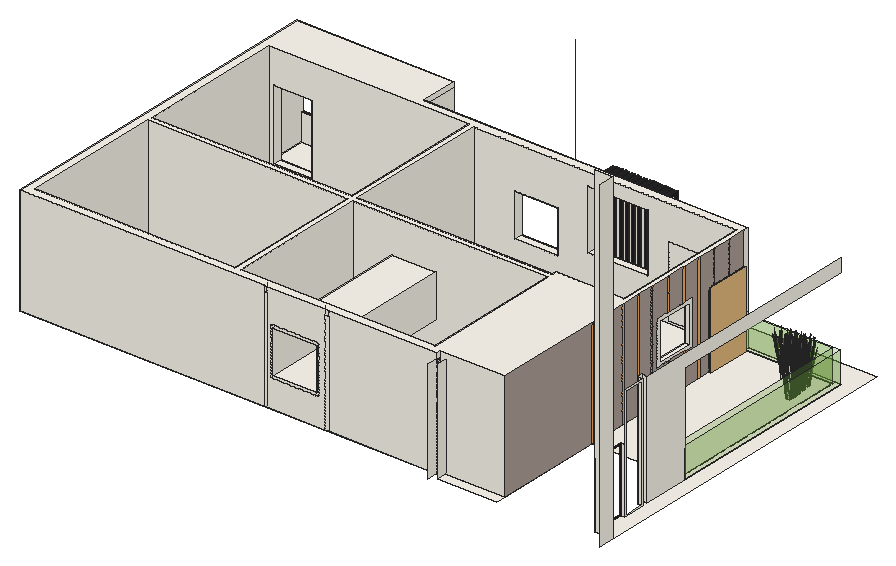
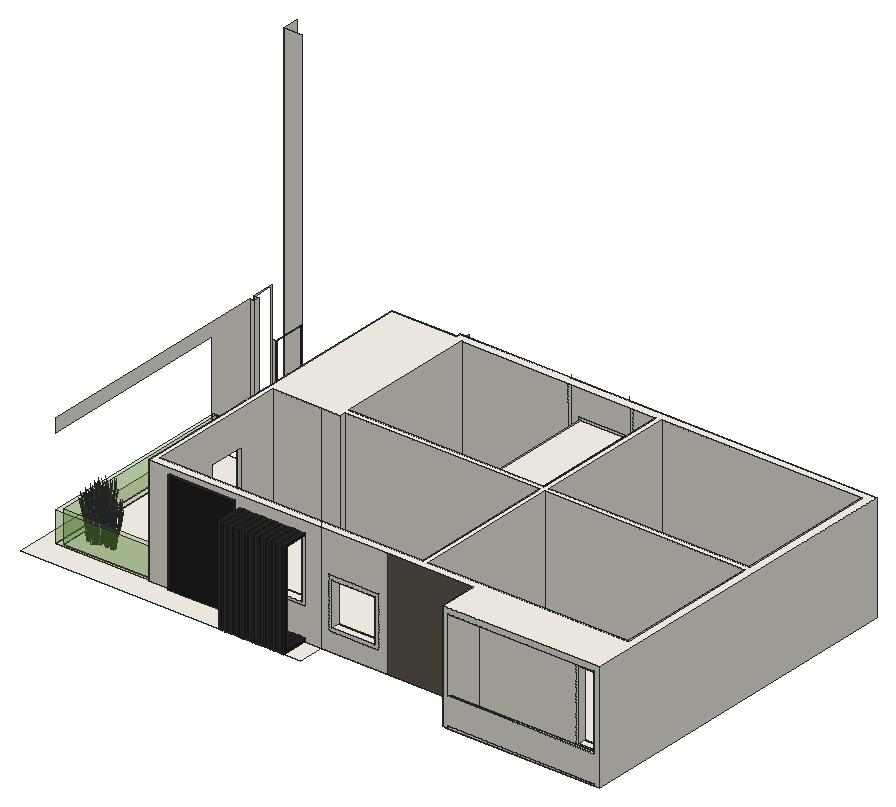
# SketchUp Ruby script. Lengths in inches.
U = 1.inch
M = Sketchup.active_model
def pt(a) = Geom::Point3d.new(a.map { |v| v * U })
def face(e, loops, mat)
  f = e.add_face(loops[0].map { |a| pt(a) })
  loops[1..].each { |l| e.add_face(l.map { |a| pt(a) }).erase! }
  f.material = f.back_material = mat if mat
  f
end
# faces: each face lists its corners as indices into pts; further lists are holes
def faces(e, pts, list, mat = nil) = list.each { |f| face(e, (f[0].is_a?(Array) ? f : [f]).map { |l| l.map { |i| pts[i] } }, mat) }
# xy, xz, yz: faces in a plane at the given z, y or x. An outline is a flat list of corners, or four numbers for a rectangle; further outlines are holes
def ring(l) = l.size == 4 ? [[l[0], l[1]], [l[2], l[1]], [l[2], l[3]], [l[0], l[3]]] : l.each_slice(2).to_a
def flat(e, list, mat, &to3) = list.each { |f| face(e, (f[0].is_a?(Array) ? f : [f]).map { |l| ring(l).map { |u, v| to3.(u, v) } }, mat) }
def xy(e, z, list, mat = nil) = flat(e, list, mat) { |x, y| [x, y, z] }
def xz(e, y, list, mat = nil) = flat(e, list, mat) { |x, z| [x, y, z] }
def yz(e, x, list, mat = nil) = flat(e, list, mat) { |y, z| [x, y, z] }
def lines(e, pts, list) = list.each { |a, b| e.add_line(pt(pts[a]), pt(pts[b])) }
# prism: a flat outline (further loops are holes) pulled along v
def prism(e, loops, v, mat = nil)
  f = face(e, loops, mat); d = Geom::Vector3d.new(v.map { |x| x * U })
  f.pushpull(f.normal.samedirection?(d) ? d.length : -d.length)
end
def box(e, o, s, mat = nil) = prism(e, [[o, [o[0] + s[0], o[1], o[2]], [o[0] + s[0], o[1] + s[1], o[2]], [o[0], o[1] + s[1], o[2]]]], [0, 0, s[2]], mat)
def at(x, y, z, deg = 0) = Geom::Transformation.translation(pt([x, y, z])) * Geom::Transformation.rotation(ORIGIN, Z_AXIS, deg.degrees)
def axes(o, x, y, z) = Geom::Transformation.new([*x, 0, *y, 0, *z, 0, *pt(o).to_a, 1])
def part(name) = M.definitions.add(name)
# library, detail: a bought-in or finely detailed component or shape, given as its bounding box
def library(name, o, s) = part(name).tap { |d| box(d.entities, o, s) }
def detail(e, o, s) = box(e.add_group.entities, o, s)
def put(e, d, t, mat = nil) = e.add_instance(d, t).tap { |i| i.material = mat if mat }
def group(e, t, mat = nil) = e.add_group.tap { |g| g.transformation = t; g.material = mat if mat }.entities
root = M.entities
M.materials.add("C01_Vanilla_Cream").color = [255, 251, 241]
M.materials.add("C03_Honey_Glow").color = [255, 178, 101]
M.materials.add("Glass_Basic_01").color = [119, 186, 61]
M.materials["Glass_Basic_01"].alpha = 0.25
M.materials.add("LightPink_Translucent").color = [144, 107, 117]
M.materials["LightPink_Translucent"].alpha = 0.75
M.materials.add("Marble_07_1K").color = [36, 34, 36]
M.materials.add("Plaster_04_1K").color = [106, 98, 87]
M.materials.add("ThomThom - Hair1").color = [178, 163, 155]
c1 = library("porta+4",[0.2,-5.42,1.33],[46.55,4.72,83.21])
c2 = part("blade")
p = [[2.15,0.21,22],[0,0.17,0],[0.09,0.45,0],[2.18,0.31,22],[2.29,0.31,22],[0.38,0.45,0],
  [2.48,0.24,33],[2.49,0.24,33],[2.48,0.22,33]]
faces(c2.entities,p,[[0,1,2,3],[4,5,2,3],[6,3,4,7],[8,0,3,6]])
c3 = part("seeds")
p = [[0.3,-0.1,1.38],[-0.01,-0.03,1.59],[-0.01,-0.03,0.03],[0.14,-0.07,-0.07],[0.29,-0.03,3],[0.15,0.01,3.11]]
faces(c3.entities,p,[[0,1,2,3],[1,0,4,5]],"LightPink_Translucent")
c4 = part("blade with seeds")
put(c4.entities,c2,at(0,0,0))
put(c4.entities,c3,axes([2.4,0.25,30.99],[1.5799,-0.05474,1.17369],[-0.12525,1.92788,0.29478],[-0.07173,-0.02425,1.56792]))
xy(root,264,[[537,12,603,24],[69,18,531,18,531,24,603,24,603,360,243,360,243,402,69,402],[702,24,722,24,722,389.16,411,389.16,411,360,706,360,706,91.21,700,91.21,700,85.38,706,85.38,706,60,702,60],[603,144,699.71,356],[699.71,144,706,360],
  [603,356,699.71,360]],"C01_Vanilla_Cream")
xz(root,24,[[531,264,537,378],[702,264,722,624]],"C01_Vanilla_Cream")
xz(root,60,[[702,264,706,336]],"C01_Vanilla_Cream")
xz(root,85.38,[[700,264,706,390]],"C01_Vanilla_Cream")
xz(root,91.21,[[700,264,706,390]],"C01_Vanilla_Cream")
xz(root,144,[[693.41,264,699.71,300],[699.71,264,706,300]],"C01_Vanilla_Cream")
xz(root,356,[[603,264,699.71,300]],"Glass_Basic_01")
xz(root,360,[[603,264,706,298]],"Glass_Basic_01")
yz(root,531,[[6,264,24,378]],"C01_Vanilla_Cream")
yz(root,537,[[12,264,24,378]],"C01_Vanilla_Cream")
yz(root,603,[[356,264,360,300]],"C01_Vanilla_Cream")
yz(root,699.71,[[144,264,356,300]],"Glass_Basic_01")
yz(root,700,[[85.38,264,91.21,390]],"C01_Vanilla_Cream")
yz(root,702,[[[24,264,60,336],[25,265,59,335]]],"Marble_07_1K")
yz(root,706,[[[60,264,85.38,390],[61,265,84.38,389]],[91.21,264,144,264,144,375,360,375,360,390,91.21,390]],"C01_Vanilla_Cream")
yz(root,706,[[144,264,360,298]],"Glass_Basic_01")
yz(root,722,[[6,264,24,624]],"C01_Vanilla_Cream")
p = [[411,360,504],[411,360,264]]
lines(root,p,[[0,1]])
put(root,c1,axes([599.84,305.79,262.64],[0,1.03118,0],[-1,0,0],[0,0,1.00971]))
g1 = group(root,at(69,18,264),"C01_Vanilla_Cream")
xy(g1,0,[[[0,0,0,384,6,384,6,342,168,342,168,384,174,384,174,342,360.88,342,360.88,371.16,364.88,371.16,364.88,342,367.67,342,367.67,371.16,371.67,371.16,371.67,342,374.46,342,374.46,371.16,378.46,371.16,378.46,342,381.25,342,381.25,371.16,385.25,371.16,385.25,342,388.04,342,388.04,371.16,392.04,371.16,392.04,342,394.83,342,394.83,371.16,398.83,371.16,398.83,342,401.62,342,401.62,371.16,405.62,371.16,405.62,342,408.41,342,408.41,371.16,412.41,371.16,412.41,342,415.2,342,415.2,371.16,419.2,371.16,419.2,342,421.99,342,421.99,371.16,425.99,371.16,425.99,342,428.77,342,428.77,371.16,432.77,371.16,432.77,342,438,342,438,344,510.88,344,510.88,342,534,342,534,4.78,462,4.78,462,0],[237,171,453,171,453,177,528.58,177,528.58,333,237,333],[9,171,231,333],[9,9,231,165]],[6,342,168,384]])
xy(g1,2,[[6,342,168,381],[6,381,168,384]])
xy(g1,3,[[528.58,291,534,333]])
xy(g1,4,[[360.88,342,364.88,367.16],[367.67,342,371.67,367.16],[374.46,342,378.46,367.16],[381.25,342,385.25,367.16],[388.04,342,392.04,367.16],
  [394.83,342,398.83,367.16],[401.62,342,405.62,367.16],[408.41,342,412.41,367.16],[415.2,342,419.2,367.16],[421.99,342,425.99,367.16],
  [428.77,342,432.77,367.16]],"Marble_07_1K")
xy(g1,5,[[15,333,57,342]])
xy(g1,24.28,[[282.48,333,330.48,342]])
xy(g1,32,[[6,381,168,384]])
xy(g1,33.28,[[280.68,0,328.68,165]])
xy(g1,39,[[528.58,219,534,261],[363.77,333,429.77,342]])
xy(g1,72.28,[[282.48,333,330.48,342]])
xy(g1,81,[[528.58,219,534,261],[528.58,291,534,333]])
xy(g1,81.28,[[280.68,0,328.68,165]])
xy(g1,83,[[15,333,57,342]])
xy(g1,105,[[363.77,333,429.77,342],[360.88,342,364.5,367.16],[364.5,342,364.88,367.16],[367.67,342,371.67,367.16],[374.46,342,378.46,367.16],
  [381.25,342,385.25,367.16],[388.04,342,392.04,367.16],[394.83,342,398.83,367.16],[401.62,342,405.62,367.16],[408.41,342,412.41,367.16],
  [415.2,342,419.2,367.16],[421.99,342,425.99,367.16],[428.77,342,432.77,367.16]])
xy(g1,108,[[360.88,342,364.88,371.16],[367.67,342,371.67,371.16],[374.46,342,378.46,371.16],[381.25,342,385.25,371.16],[388.04,342,392.04,371.16],
  [394.83,342,398.83,371.16],[401.62,342,405.62,371.16],[408.41,342,412.41,371.16],[415.2,342,419.2,371.16],[421.99,342,425.99,371.16],
  [428.77,342,432.77,371.16]],"Marble_07_1K")
xy(g1,114,[[6,342,168,384]])
xy(g1,114,[[438,342,510.88,344]],"Marble_07_1K")
xy(g1,120,[[[0,0,462,0,462,4.78,534,4.78,534,342,174,342,174,384,0,384],[237,171,237,333,528.58,333,528.58,177,453,177,453,171],[9,171,231,333],[9,9,231,165],[237,9,453,165]]])
xz(g1,0,[[0,0,270,120],[270,0,274,114],[[274,0,338,120],[277.68,30.28,331.68,84.28]],[338,0,342,114],[342,0,462,120],
  [[277.68,30.28,331.68,84.28],[280.68,33.28,328.68,81.28]],[270,114,274,120],[338,114,342,120]])
xz(g1,4.78,[[462,0,534,120]])
xz(g1,9,[[9,0,231,120]])
xz(g1,165,[[9,0,231,120],[[237,0,453,120],[280.68,33.28,328.68,81.28]]])
xz(g1,171,[[9,0,231,120],[237,0,453,120]])
xz(g1,177,[[453,0,528.58,120]])
xz(g1,219,[[528.58,39,534,81]])
xz(g1,261,[[528.58,39,534,81]])
xz(g1,291,[[528.58,3,534,81]])
xz(g1,333,[[[9,0,231,120],[15,5,57,83]],[[237,0,528.58,0,528.58,3,453,3,453,81,528.58,81,528.58,120,237,120],[363.77,39,429.77,105],[282.48,24.28,330.48,72.28]],[453,3,534,81]])
xz(g1,342,[[6,0,168,2],[[270,0,270,120,534,120,534,0,510.88,0,510.88,114,438,114,438,0,432.77,0,432.77,4,428.77,4,428.77,0,425.99,0,425.99,4,421.99,4,421.99,0,419.2,0,419.2,4,415.2,4,415.2,0,412.41,0,412.41,4,408.41,4,408.41,0,405.62,0,405.62,4,401.62,4,401.62,0,398.83,0,398.83,4,394.83,4,394.83,0,392.04,0,392.04,4,388.04,4,388.04,0,385.25,0,385.25,4,381.25,4,381.25,0,378.46,0,378.46,4,374.46,4,374.46,0,371.67,0,371.67,4,367.67,4,367.67,0,364.88,0,364.88,4,360.88,4,360.88,0,360.77,0,360.77,36,432.77,36,432.77,108,360.77,108,360.77,0],[278.48,20.28,334.48,76.28]],[[12,2,60,86],[15,5,57,83]],[[278.48,20.28,334.48,76.28],[282.48,24.28,330.48,72.28]],[360.77,36,360.77,108,360.88,108,360.88,105,363.77,105,363.77,39,429.77,39,429.77,105,432.77,105,432.77,36],
  [360.88,105,364.88,108],[364.88,105,367.67,108],[367.67,105,371.67,108],[371.67,105,374.46,108],[374.46,105,378.46,108],
  [378.46,105,381.25,108],[381.25,105,385.25,108],[385.25,105,388.04,108],[388.04,105,392.04,108],[392.04,105,394.83,108],
  [394.83,105,398.83,108],[398.83,105,401.62,108],[401.62,105,405.62,108],[405.62,105,408.41,108],[408.41,105,412.41,108],
  [412.41,105,415.2,108],[415.2,105,419.2,108],[419.2,105,421.99,108],[421.99,105,425.99,108],[425.99,105,428.77,108],
  [428.77,105,432.77,108]])
xz(g1,342,[[6,2,6,114,168,114,168,2,60,2,60,86,12,86,12,2]],"C01_Vanilla_Cream")
xz(g1,342,[[174,0,270,120]],"Plaster_04_1K")
xz(g1,344,[[438,0,510.88,114]],"Marble_07_1K")
xz(g1,367.16,[[360.88,4,364.5,105],[364.5,4,364.88,105],[367.67,4,371.67,105],[374.46,4,378.46,105],[381.25,4,385.25,105],
  [388.04,4,392.04,105],[394.83,4,398.83,105],[401.62,4,405.62,105],[408.41,4,412.41,105],[415.2,4,419.2,105],
  [421.99,4,425.99,105],[428.77,4,432.77,105]])
xz(g1,371.16,[[360.88,0,364.88,108],[367.67,0,371.67,108],[374.46,0,378.46,108],[381.25,0,385.25,108],[388.04,0,392.04,108],
  [394.83,0,398.83,108],[401.62,0,405.62,108],[408.41,0,412.41,108],[415.2,0,419.2,108],[421.99,0,425.99,108],
  [428.77,0,432.77,108]],"Marble_07_1K")
xz(g1,381,[[6,2,168,32]])
xz(g1,384,[[[0,0,0,120,174,120,174,0,168,0,168,2,6,2,6,0],[6,32,168,114]],[6,0,168,2]])
yz(g1,0,[[0,0,384,120]])
yz(g1,6,[[342,0,384,2],[342,2,381,2,381,32,384,32,384,114,342,114]])
yz(g1,9,[[9,0,165,120],[171,0,333,120]])
yz(g1,15,[[333,5,342,83]])
yz(g1,57,[[333,5,342,83]])
yz(g1,168,[[342,0,384,2],[342,2,342,114,384,114,384,32,381,32,381,2]])
yz(g1,174,[[342,0,384,114],[342,114,384,120]])
yz(g1,231,[[9,0,165,120],[171,0,333,120]])
yz(g1,237,[[9,0,165,120],[171,0,333,120]])
yz(g1,280.68,[[0,33.28,165,81.28]])
yz(g1,282.48,[[333,24.28,342,72.28]])
yz(g1,328.68,[[0,33.28,165,81.28]])
yz(g1,330.48,[[333,24.28,342,72.28]])
yz(g1,360.88,[[342,0,342,4,367.16,4,367.16,105,342,105,342,108,371.16,108,371.16,0]],"Marble_07_1K")
yz(g1,363.77,[[333,39,342,105]])
yz(g1,364.88,[[342,0,371.16,0,371.16,108,342,108,342,105,367.16,105,367.16,4,342,4]],"Marble_07_1K")
yz(g1,367.67,[[342,0,342,4,367.16,4,367.16,105,342,105,342,108,371.16,108,371.16,0]],"Marble_07_1K")
yz(g1,371.67,[[342,0,371.16,0,371.16,108,342,108,342,105,367.16,105,367.16,4,342,4]],"Marble_07_1K")
yz(g1,374.46,[[342,0,342,4,367.16,4,367.16,105,342,105,342,108,371.16,108,371.16,0]],"Marble_07_1K")
yz(g1,378.46,[[342,0,371.16,0,371.16,108,342,108,342,105,367.16,105,367.16,4,342,4]],"Marble_07_1K")
yz(g1,381.25,[[342,0,342,4,367.16,4,367.16,105,342,105,342,108,371.16,108,371.16,0]],"Marble_07_1K")
yz(g1,385.25,[[342,0,371.16,0,371.16,108,342,108,342,105,367.16,105,367.16,4,342,4]],"Marble_07_1K")
yz(g1,388.04,[[342,0,342,4,367.16,4,367.16,105,342,105,342,108,371.16,108,371.16,0]],"Marble_07_1K")
yz(g1,392.04,[[342,0,371.16,0,371.16,108,342,108,342,105,367.16,105,367.16,4,342,4]],"Marble_07_1K")
yz(g1,394.83,[[342,0,342,4,367.16,4,367.16,105,342,105,342,108,371.16,108,371.16,0]],"Marble_07_1K")
yz(g1,398.83,[[342,0,371.16,0,371.16,108,342,108,342,105,367.16,105,367.16,4,342,4]],"Marble_07_1K")
yz(g1,401.62,[[342,0,342,4,367.16,4,367.16,105,342,105,342,108,371.16,108,371.16,0]],"Marble_07_1K")
yz(g1,405.62,[[342,0,371.16,0,371.16,108,342,108,342,105,367.16,105,367.16,4,342,4]],"Marble_07_1K")
yz(g1,408.41,[[342,0,342,4,367.16,4,367.16,105,342,105,342,108,371.16,108,371.16,0]],"Marble_07_1K")
yz(g1,412.41,[[342,0,371.16,0,371.16,108,342,108,342,105,367.16,105,367.16,4,342,4]],"Marble_07_1K")
yz(g1,415.2,[[342,0,342,4,367.16,4,367.16,105,342,105,342,108,371.16,108,371.16,0]],"Marble_07_1K")
yz(g1,419.2,[[342,0,371.16,0,371.16,108,342,108,342,105,367.16,105,367.16,4,342,4]],"Marble_07_1K")
yz(g1,421.99,[[342,0,342,4,367.16,4,367.16,105,342,105,342,108,371.16,108,371.16,0]],"Marble_07_1K")
yz(g1,425.99,[[342,0,371.16,0,371.16,108,342,108,342,105,367.16,105,367.16,4,342,4]],"Marble_07_1K")
yz(g1,428.77,[[342,0,342,4,367.16,4,367.16,105,342,105,342,108,371.16,108,371.16,0]],"Marble_07_1K")
yz(g1,429.77,[[333,39,342,55.56],[333,55.56,342,105]])
yz(g1,432.77,[[342,0,371.16,0,371.16,108,342,108,342,105,367.16,105,367.16,4,342,4]],"Marble_07_1K")
yz(g1,438,[[342,0,344,114]],"Marble_07_1K")
yz(g1,453,[[9,0,165,120],[171,0,177,120]])
yz(g1,462,[[0,0,4.78,120]])
yz(g1,510.88,[[342,0,344,114]],"Marble_07_1K")
yz(g1,528.58,[[[177,0,177,120,333,120,333,81,291,81,291,3,333,3,333,0],[219,39,261,81]]])
yz(g1,534,[[[288,0,336,84],[291,3,333,81]],[336,0,342,120],[[216,36,264,84],[219,39,261,81]]])
yz(g1,534,[[125.4,0,127.4,120],[146.46,0,148.46,120],[167.52,0,169.52,120],[188.58,0,190.58,120],[207.64,0,209.64,120],
  [230.7,0,232.7,36],[251.76,0,253.76,36],[272.82,0,274.82,120],[230.7,84,232.7,120],[251.76,84,253.76,120],
  [293.88,84,295.88,120],[314.94,84,316.94,120]],"C03_Honey_Glow")
yz(g1,534,[[4.78,0,125.4,120],[127.4,0,146.46,120],[148.46,0,167.52,120],[169.52,0,188.58,120],[190.58,0,207.64,120],
  [209.64,0,230.7,0,230.7,36,216,36,216,84,230.7,84,230.7,120,209.64,120],[232.7,0,251.76,36],[253.76,0,272.82,0,272.82,120,253.76,120,253.76,84,264,84,264,36,253.76,36],[274.82,0,288,0,288,84,293.88,84,293.88,120,274.82,120],[232.7,84,251.76,120],
  [295.88,84,314.94,120],[316.94,84,336,120]],"ThomThom - Hair1")
p = [[274,0,124],[274,0,120],[338,0,124],[338,0,120]]
lines(g1,p,[[0,1],[2,3]])
put(root,c4,axes([659.37,336.51,265.74],[-0.26718,-0.5855,-0.57963],[0.76964,-0.21087,-0.15213],[-0.02953,-0.19827,1.27944]))
put(root,c4,axes([666.07,335.97,265.74],[-0.26718,-0.5855,-0.57963],[0.76964,-0.21087,-0.15213],[-0.02953,-0.19827,1.27944]))
put(root,c4,axes([673.97,336.56,265.74],[-0.26718,-0.5855,-0.57963],[0.76964,-0.21087,-0.15213],[-0.02953,-0.19827,1.27944]))
put(root,c4,axes([678.77,339.64,265.74],[-0.26718,-0.5855,-0.57963],[0.76964,-0.21087,-0.15213],[-0.02953,-0.19827,1.27944]))
put(root,c4,axes([684.2,338.09,265.74],[-0.26718,-0.5855,-0.57963],[0.76964,-0.21087,-0.15213],[-0.02953,-0.19827,1.27944]))
put(root,c4,axes([685.54,329.9,265.74],[-0.26718,-0.5855,-0.57963],[0.76964,-0.21087,-0.15213],[-0.02953,-0.19827,1.27944]))
put(root,c4,axes([686.59,321.7,265.74],[-0.26718,-0.5855,-0.57963],[0.76964,-0.21087,-0.15213],[-0.02953,-0.19827,1.27944]))
put(root,c4,axes([687.05,315.16,265.74],[-0.26718,-0.5855,-0.57963],[0.76964,-0.21087,-0.15213],[-0.02953,-0.19827,1.27944]))
put(root,c4,axes([686.625,310.22,265.74],[-0.26718,-0.5855,-0.57963],[0.76964,-0.21087,-0.15213],[-0.02953,-0.19827,1.27944]))
put(root,c4,axes([661.81,337.5,265.74],[0.23855,0.52277,-0.57446],[-0.68718,0.18827,-0.15077],[0.02637,0.17702,1.26801]))
put(root,c4,axes([668.51,336.96,265.74],[0.23855,0.52277,-0.57446],[-0.68718,0.18827,-0.15077],[0.02637,0.17702,1.26801]))
put(root,c4,axes([676.41,337.56,265.74],[0.23855,0.52277,-0.57446],[-0.68718,0.18827,-0.15077],[0.02637,0.17702,1.26801]))
put(root,c4,axes([681.21,340.63,265.74],[0.23855,0.52277,-0.57446],[-0.68718,0.18827,-0.15077],[0.02637,0.17702,1.26801]))
put(root,c4,axes([686.64,339.09,265.74],[0.23855,0.52277,-0.57446],[-0.68718,0.18827,-0.15077],[0.02637,0.17702,1.26801]))
put(root,c4,axes([687.98,330.9,265.74],[0.23855,0.52277,-0.57446],[-0.68718,0.18827,-0.15077],[0.02637,0.17702,1.26801]))
put(root,c4,axes([689.03,322.7,265.74],[0.23855,0.52277,-0.57446],[-0.68718,0.18827,-0.15077],[0.02637,0.17702,1.26801]))
put(root,c4,axes([689.49,316.16,265.74],[0.23855,0.52277,-0.57446],[-0.68718,0.18827,-0.15077],[0.02637,0.17702,1.26801]))
put(root,c4,axes([689.07,311.22,265.74],[0.23855,0.52277,-0.57446],[-0.68718,0.18827,-0.15077],[0.02637,0.17702,1.26801]))
put(root,c4,axes([661.74,336.4,265.71],[0.67676,0.09361,-0.51753],[-0.14281,0.57742,-0.13583],[0.20196,0.06997,1.14236]))
put(root,c4,axes([659.47,337.6,265.71],[-0.67676,-0.09361,-0.51753],[0.14281,-0.57742,-0.13583],[-0.20196,-0.06997,1.14236]))
put(root,c4,axes([660.54,335.9,265.71],[0.43821,-0.42916,-0.51753],[0.54436,0.38915,-0.13583],[0.1756,-0.10706,1.14236]))
put(root,c4,axes([660.67,338.1,265.71],[-0.43821,0.42916,-0.51753],[-0.54436,-0.38915,-0.13583],[-0.1756,0.10706,1.14236]))
put(root,c4,axes([668.44,335.87,265.71],[0.67676,0.09361,-0.51753],[-0.14281,0.57742,-0.13583],[0.20196,0.06997,1.14236]))
put(root,c4,axes([666.17,337.0625,265.71],[-0.67676,-0.09361,-0.51753],[0.14281,-0.57742,-0.13583],[-0.20196,-0.06997,1.14236]))
put(root,c4,axes([667.24,335.37,265.71],[0.43821,-0.42916,-0.51753],[0.54436,0.38915,-0.13583],[0.1756,-0.10706,1.14236]))
put(root,c4,axes([667.38,337.5625,265.71],[-0.43821,0.42916,-0.51753],[-0.54436,-0.38915,-0.13583],[-0.1756,0.10706,1.14236]))
put(root,c4,axes([676.34,336.46,265.71],[0.67676,0.09361,-0.51753],[-0.14281,0.57742,-0.13583],[0.20196,0.06997,1.14236]))
put(root,c4,axes([674.08,337.66,265.71],[-0.67676,-0.09361,-0.51753],[0.14281,-0.57742,-0.13583],[-0.20196,-0.06997,1.14236]))
put(root,c4,axes([675.14,335.96,265.71],[0.43821,-0.42916,-0.51753],[0.54436,0.38915,-0.13583],[0.1756,-0.10706,1.14236]))
put(root,c4,axes([675.28,338.16,265.71],[-0.43821,0.42916,-0.51753],[-0.54436,-0.38915,-0.13583],[-0.1756,0.10706,1.14236]))
put(root,c4,axes([681.15,339.53,265.71],[0.67676,0.09361,-0.51753],[-0.14281,0.57742,-0.13583],[0.20196,0.06997,1.14236]))
put(root,c4,axes([678.875,340.73,265.71],[-0.67676,-0.09361,-0.51753],[0.14281,-0.57742,-0.13583],[-0.20196,-0.06997,1.14236]))
put(root,c4,axes([679.94,339.03,265.71],[0.43821,-0.42916,-0.51753],[0.54436,0.38915,-0.13583],[0.1756,-0.10706,1.14236]))
put(root,c4,axes([680.08,341.23,265.71],[-0.43821,0.42916,-0.51753],[-0.54436,-0.38915,-0.13583],[-0.1756,0.10706,1.14236]))
put(root,c4,axes([686.57,337.99,265.71],[0.67676,0.09361,-0.51753],[-0.14281,0.57742,-0.13583],[0.20196,0.06997,1.14236]))
put(root,c4,axes([684.3,339.19,265.71],[-0.67676,-0.09361,-0.51753],[0.14281,-0.57742,-0.13583],[-0.20196,-0.06997,1.14236]))
put(root,c4,axes([685.37,337.49,265.71],[0.43821,-0.42916,-0.51753],[0.54436,0.38915,-0.13583],[0.1756,-0.10706,1.14236]))
put(root,c4,axes([685.51,339.68,265.71],[-0.43821,0.42916,-0.51753],[-0.54436,-0.38915,-0.13583],[-0.1756,0.10706,1.14236]))
put(root,c4,axes([687.91,329.8,265.71],[0.67676,0.09361,-0.51753],[-0.14281,0.57742,-0.13583],[0.20196,0.06997,1.14236]))
put(root,c4,axes([685.64,331,265.71],[-0.67676,-0.09361,-0.51753],[0.14281,-0.57742,-0.13583],[-0.20196,-0.06997,1.14236]))
put(root,c4,axes([686.71,329.3,265.71],[0.43821,-0.42916,-0.51753],[0.54436,0.38915,-0.13583],[0.1756,-0.10706,1.14236]))
put(root,c4,axes([686.85,331.5,265.71],[-0.43821,0.42916,-0.51753],[-0.54436,-0.38915,-0.13583],[-0.1756,0.10706,1.14236]))
put(root,c4,axes([688.97,321.6,265.71],[0.67676,0.09361,-0.51753],[-0.14281,0.57742,-0.13583],[0.20196,0.06997,1.14236]))
put(root,c4,axes([686.7,322.8,265.71],[-0.67676,-0.09361,-0.51753],[0.14281,-0.57742,-0.13583],[-0.20196,-0.06997,1.14236]))
put(root,c4,axes([687.76,321.1,265.71],[0.43821,-0.42916,-0.51753],[0.54436,0.38915,-0.13583],[0.1756,-0.10706,1.14236]))
put(root,c4,axes([687.9,323.3,265.71],[-0.43821,0.42916,-0.51753],[-0.54436,-0.38915,-0.13583],[-0.1756,0.10706,1.14236]))
put(root,c4,axes([689.42,315.0625,265.71],[0.67676,0.09361,-0.51753],[-0.14281,0.57742,-0.13583],[0.20196,0.06997,1.14236]))
put(root,c4,axes([687.15,316.26,265.71],[-0.67676,-0.09361,-0.51753],[0.14281,-0.57742,-0.13583],[-0.20196,-0.06997,1.14236]))
put(root,c4,axes([688.22,314.5625,265.71],[0.43821,-0.42916,-0.51753],[0.54436,0.38915,-0.13583],[0.1756,-0.10706,1.14236]))
put(root,c4,axes([688.36,316.76,265.71],[-0.43821,0.42916,-0.51753],[-0.54436,-0.38915,-0.13583],[-0.1756,0.10706,1.14236]))
put(root,c4,axes([689,310.12,265.71],[0.67676,0.09361,-0.51753],[-0.14281,0.57742,-0.13583],[0.20196,0.06997,1.14236]))
put(root,c4,axes([686.73,311.3125,265.71],[-0.67676,-0.09361,-0.51753],[0.14281,-0.57742,-0.13583],[-0.20196,-0.06997,1.14236]))
put(root,c4,axes([687.8,309.62,265.71],[0.43821,-0.42916,-0.51753],[0.54436,0.38915,-0.13583],[0.1756,-0.10706,1.14236]))
put(root,c4,axes([687.93,311.8125,265.71],[-0.43821,0.42916,-0.51753],[-0.54436,-0.38915,-0.13583],[-0.1756,0.10706,1.14236]))
put(root,c4,axes([662.63,335.31,265.67],[0.60889,0.28548,-0.4121],[-0.36394,0.51192,0],[0.13868,0.06502,1.30728]))
put(root,c4,axes([661.4,339.27,265.67],[-0.60889,0.28548,-0.4121],[-0.36394,-0.51192,0],[-0.13868,0.06502,1.30728]))
put(root,c4,axes([657.79,336.42,265.67],[0,-0.57097,-0.4121],[0.72788,0,0],[0,-0.13004,1.30728]))
put(root,c4,axes([658.58,338.69,265.67],[-0.60889,-0.28548,-0.4121],[0.36394,-0.51192,0],[-0.13868,-0.06502,1.30728]))
put(root,c4,axes([659.8125,334.73,265.67],[0.60889,-0.28548,-0.4121],[0.36394,0.51192,0],[0.13868,-0.06502,1.30728]))
put(root,c4,axes([663.42,337.58,265.67],[0,0.57097,-0.4121],[-0.72788,0,0],[0,0.13004,1.30728]))
put(root,c4,axes([669.33,334.78,265.67],[0.60889,0.28548,-0.4121],[-0.36394,0.51192,0],[0.13868,0.06502,1.30728]))
put(root,c4,axes([668.1,338.73,265.67],[-0.60889,0.28548,-0.4121],[-0.36394,-0.51192,0],[-0.13868,0.06502,1.30728]))
put(root,c4,axes([664.5,335.89,265.67],[0,-0.57097,-0.4121],[0.72788,0,0],[0,-0.13004,1.30728]))
put(root,c4,axes([665.29,338.16,265.67],[-0.60889,-0.28548,-0.4121],[0.36394,-0.51192,0],[-0.13868,-0.06502,1.30728]))
put(root,c4,axes([666.52,334.2,265.67],[0.60889,-0.28548,-0.4121],[0.36394,0.51192,0],[0.13868,-0.06502,1.30728]))
put(root,c4,axes([670.125,337.04,265.67],[0,0.57097,-0.4121],[-0.72788,0,0],[0,0.13004,1.30728]))
put(root,c4,axes([677.23,335.37,265.67],[0.60889,0.28548,-0.4121],[-0.36394,0.51192,0],[0.13868,0.06502,1.30728]))
put(root,c4,axes([676,339.33,265.67],[-0.60889,0.28548,-0.4121],[-0.36394,-0.51192,0],[-0.13868,0.06502,1.30728]))
put(root,c4,axes([672.4,336.48,265.67],[0,-0.57097,-0.4121],[0.72788,0,0],[0,-0.13004,1.30728]))
put(root,c4,axes([673.1875,338.75,265.67],[-0.60889,-0.28548,-0.4121],[0.36394,-0.51192,0],[-0.13868,-0.06502,1.30728]))
put(root,c4,axes([674.42,334.79,265.67],[0.60889,-0.28548,-0.4121],[0.36394,0.51192,0],[0.13868,-0.06502,1.30728]))
put(root,c4,axes([678.02,337.64,265.67],[0,0.57097,-0.4121],[-0.72788,0,0],[0,0.13004,1.30728]))
put(root,c4,axes([682.03,338.44,265.67],[0.60889,0.28548,-0.4121],[-0.36394,0.51192,0],[0.13868,0.06502,1.30728]))
put(root,c4,axes([680.8,342.4,265.67],[-0.60889,0.28548,-0.4121],[-0.36394,-0.51192,0],[-0.13868,0.06502,1.30728]))
put(root,c4,axes([677.2,339.55,265.67],[0,-0.57097,-0.4121],[0.72788,0,0],[0,-0.13004,1.30728]))
put(root,c4,axes([677.99,341.82,265.67],[-0.60889,-0.28548,-0.4121],[0.36394,-0.51192,0],[-0.13868,-0.06502,1.30728]))
put(root,c4,axes([679.22,337.86,265.67],[0.60889,-0.28548,-0.4121],[0.36394,0.51192,0],[0.13868,-0.06502,1.30728]))
put(root,c4,axes([682.82,340.71,265.67],[0,0.57097,-0.4121],[-0.72788,0,0],[0,0.13004,1.30728]))
put(root,c4,axes([687.46,336.9,265.67],[0.60889,0.28548,-0.4121],[-0.36394,0.51192,0],[0.13868,0.06502,1.30728]))
put(root,c4,axes([686.23,340.86,265.67],[-0.60889,0.28548,-0.4121],[-0.36394,-0.51192,0],[-0.13868,0.06502,1.30728]))
put(root,c4,axes([682.62,338.01,265.67],[0,-0.57097,-0.4121],[0.72788,0,0],[0,-0.13004,1.30728]))
put(root,c4,axes([683.41,340.28,265.67],[-0.60889,-0.28548,-0.4121],[0.36394,-0.51192,0],[-0.13868,-0.06502,1.30728]))
put(root,c4,axes([684.65,336.32,265.67],[0.60889,-0.28548,-0.4121],[0.36394,0.51192,0],[0.13868,-0.06502,1.30728]))
put(root,c4,axes([688.25,339.17,265.67],[0,0.57097,-0.4121],[-0.72788,0,0],[0,0.13004,1.30728]))
put(root,c4,axes([688.8,328.71,265.67],[0.60889,0.28548,-0.4121],[-0.36394,0.51192,0],[0.13868,0.06502,1.30728]))
put(root,c4,axes([687.57,332.67,265.67],[-0.60889,0.28548,-0.4121],[-0.36394,-0.51192,0],[-0.13868,0.06502,1.30728]))
put(root,c4,axes([683.96,329.82,265.67],[0,-0.57097,-0.4121],[0.72788,0,0],[0,-0.13004,1.30728]))
put(root,c4,axes([684.75,332.09,265.67],[-0.60889,-0.28548,-0.4121],[0.36394,-0.51192,0],[-0.13868,-0.06502,1.30728]))
put(root,c4,axes([685.98,328.13,265.67],[0.60889,-0.28548,-0.4121],[0.36394,0.51192,0],[0.13868,-0.06502,1.30728]))
put(root,c4,axes([689.59,330.98,265.67],[0,0.57097,-0.4121],[-0.72788,0,0],[0,0.13004,1.30728]))
put(root,c4,axes([689.85,320.51,265.67],[0.60889,0.28548,-0.4121],[-0.36394,0.51192,0],[0.13868,0.06502,1.30728]))
put(root,c4,axes([688.62,324.47,265.67],[-0.60889,0.28548,-0.4121],[-0.36394,-0.51192,0],[-0.13868,0.06502,1.30728]))
put(root,c4,axes([685.02,321.62,265.67],[0,-0.57097,-0.4121],[0.72788,0,0],[0,-0.13004,1.30728]))
put(root,c4,axes([685.81,323.89,265.67],[-0.60889,-0.28548,-0.4121],[0.36394,-0.51192,0],[-0.13868,-0.06502,1.30728]))
put(root,c4,axes([687.04,319.93,265.67],[0.60889,-0.28548,-0.4121],[0.36394,0.51192,0],[0.13868,-0.06502,1.30728]))
put(root,c4,axes([690.64,322.78,265.67],[0,0.57097,-0.4121],[-0.72788,0,0],[0,0.13004,1.30728]))
put(root,c4,axes([690.31,313.97,265.67],[0.60889,0.28548,-0.4121],[-0.36394,0.51192,0],[0.13868,0.06502,1.30728]))
put(root,c4,axes([689.08,317.93,265.67],[-0.60889,0.28548,-0.4121],[-0.36394,-0.51192,0],[-0.13868,0.06502,1.30728]))
put(root,c4,axes([685.47,315.08,265.67],[0,-0.57097,-0.4121],[0.72788,0,0],[0,-0.13004,1.30728]))
put(root,c4,axes([686.26,317.35,265.67],[-0.60889,-0.28548,-0.4121],[0.36394,-0.51192,0],[-0.13868,-0.06502,1.30728]))
put(root,c4,axes([687.5,313.39,265.67],[0.60889,-0.28548,-0.4121],[0.36394,0.51192,0],[0.13868,-0.06502,1.30728]))
put(root,c4,axes([691.1,316.24,265.67],[0,0.57097,-0.4121],[-0.72788,0,0],[0,0.13004,1.30728]))
put(root,c4,axes([689.89,309.03,265.67],[0.60889,0.28548,-0.4121],[-0.36394,0.51192,0],[0.13868,0.06502,1.30728]))
put(root,c4,axes([688.66,312.98,265.67],[-0.60889,0.28548,-0.4121],[-0.36394,-0.51192,0],[-0.13868,0.06502,1.30728]))
put(root,c4,axes([685.05,310.14,265.67],[0,-0.57097,-0.4121],[0.72788,0,0],[0,-0.13004,1.30728]))
put(root,c4,axes([685.84,312.41,265.67],[-0.60889,-0.28548,-0.4121],[0.36394,-0.51192,0],[-0.13868,-0.06502,1.30728]))
put(root,c4,axes([687.07,308.45,265.67],[0.60889,-0.28548,-0.4121],[0.36394,0.51192,0],[0.13868,-0.06502,1.30728]))
put(root,c4,axes([690.68,311.29,265.67],[0,0.57097,-0.4121],[-0.72788,0,0],[0,0.13004,1.30728]))
put(root,c4,axes([659.77,336.66,265.83],[0.31565,-0.51449,-0.37133],[0.65588,0.24761,0.17871],[0,-0.1186,1.19224]))
put(root,c4,axes([659.82,337.41,265.83],[-0.39083,-0.47924,-0.37133],[0.59199,-0.33747,0.17871],[-0.12647,-0.0593,1.19224]))
put(root,c4,axes([661.39,336.59,265.83],[0.39083,0.47924,-0.37133],[-0.59199,0.33747,0.17871],[0.12647,0.0593,1.19224]))
put(root,c4,axes([661.4375,337.34,265.83],[-0.31565,0.51449,-0.37133],[-0.65588,-0.24761,0.17871],[0,0.1186,1.19224]))
put(root,c4,axes([660.65,337.76,265.83],[-0.70648,0.03525,-0.37133],[-0.06389,-0.58508,0.17871],[-0.12647,0.0593,1.19224]))
put(root,c4,axes([666.48,336.12,265.83],[0.31565,-0.51449,-0.37133],[0.65588,0.24761,0.17871],[0,-0.1186,1.19224]))
put(root,c4,axes([666.53,336.88,265.83],[-0.39083,-0.47924,-0.37133],[0.59199,-0.33747,0.17871],[-0.12647,-0.0593,1.19224]))
put(root,c4,axes([668.09,336.05,265.83],[0.39083,0.47924,-0.37133],[-0.59199,0.33747,0.17871],[0.12647,0.0593,1.19224]))
put(root,c4,axes([668.14,336.81,265.83],[-0.31565,0.51449,-0.37133],[-0.65588,-0.24761,0.17871],[0,0.1186,1.19224]))
put(root,c4,axes([667.36,337.22,265.83],[-0.70648,0.03525,-0.37133],[-0.06389,-0.58508,0.17871],[-0.12647,0.0593,1.19224]))
put(root,c4,axes([674.38,336.72,265.83],[0.31565,-0.51449,-0.37133],[0.65588,0.24761,0.17871],[0,-0.1186,1.19224]))
put(root,c4,axes([674.43,337.47,265.83],[-0.39083,-0.47924,-0.37133],[0.59199,-0.33747,0.17871],[-0.12647,-0.0593,1.19224]))
put(root,c4,axes([675.99,336.65,265.83],[0.39083,0.47924,-0.37133],[-0.59199,0.33747,0.17871],[0.12647,0.0593,1.19224]))
put(root,c4,axes([676.04,337.4,265.83],[-0.31565,0.51449,-0.37133],[-0.65588,-0.24761,0.17871],[0,0.1186,1.19224]))
put(root,c4,axes([675.26,337.82,265.83],[-0.70648,0.03525,-0.37133],[-0.06389,-0.58508,0.17871],[-0.12647,0.0593,1.19224]))
put(root,c4,axes([679.18,339.79,265.83],[0.31565,-0.51449,-0.37133],[0.65588,0.24761,0.17871],[0,-0.1186,1.19224]))
put(root,c4,axes([679.23,340.54,265.83],[-0.39083,-0.47924,-0.37133],[0.59199,-0.33747,0.17871],[-0.12647,-0.0593,1.19224]))
put(root,c4,axes([680.79,339.72,265.83],[0.39083,0.47924,-0.37133],[-0.59199,0.33747,0.17871],[0.12647,0.0593,1.19224]))
put(root,c4,axes([680.84,340.48,265.83],[-0.31565,0.51449,-0.37133],[-0.65588,-0.24761,0.17871],[0,0.1186,1.19224]))
put(root,c4,axes([680.06,340.89,265.83],[-0.70648,0.03525,-0.37133],[-0.06389,-0.58508,0.17871],[-0.12647,0.0593,1.19224]))
put(root,c4,axes([684.6,338.24,265.83],[0.31565,-0.51449,-0.37133],[0.65588,0.24761,0.17871],[0,-0.1186,1.19224]))
put(root,c4,axes([684.65,339,265.83],[-0.39083,-0.47924,-0.37133],[0.59199,-0.33747,0.17871],[-0.12647,-0.0593,1.19224]))
put(root,c4,axes([686.22,338.17,265.83],[0.39083,0.47924,-0.37133],[-0.59199,0.33747,0.17871],[0.12647,0.0593,1.19224]))
put(root,c4,axes([686.27,338.93,265.83],[-0.31565,0.51449,-0.37133],[-0.65588,-0.24761,0.17871],[0,0.1186,1.19224]))
put(root,c4,axes([685.49,339.35,265.83],[-0.70648,0.03525,-0.37133],[-0.06389,-0.58508,0.17871],[-0.12647,0.0593,1.19224]))
put(root,c4,axes([685.94,330.06,265.83],[0.31565,-0.51449,-0.37133],[0.65588,0.24761,0.17871],[0,-0.1186,1.19224]))
put(root,c4,axes([685.99,330.8125,265.83],[-0.39083,-0.47924,-0.37133],[0.59199,-0.33747,0.17871],[-0.12647,-0.0593,1.19224]))
put(root,c4,axes([687.56,329.99,265.83],[0.39083,0.47924,-0.37133],[-0.59199,0.33747,0.17871],[0.12647,0.0593,1.19224]))
put(root,c4,axes([687.61,330.74,265.83],[-0.31565,0.51449,-0.37133],[-0.65588,-0.24761,0.17871],[0,0.1186,1.19224]))
put(root,c4,axes([686.83,331.16,265.83],[-0.70648,0.03525,-0.37133],[-0.06389,-0.58508,0.17871],[-0.12647,0.0593,1.19224]))
put(root,c4,axes([687,321.86,265.83],[0.31565,-0.51449,-0.37133],[0.65588,0.24761,0.17871],[0,-0.1186,1.19224]))
